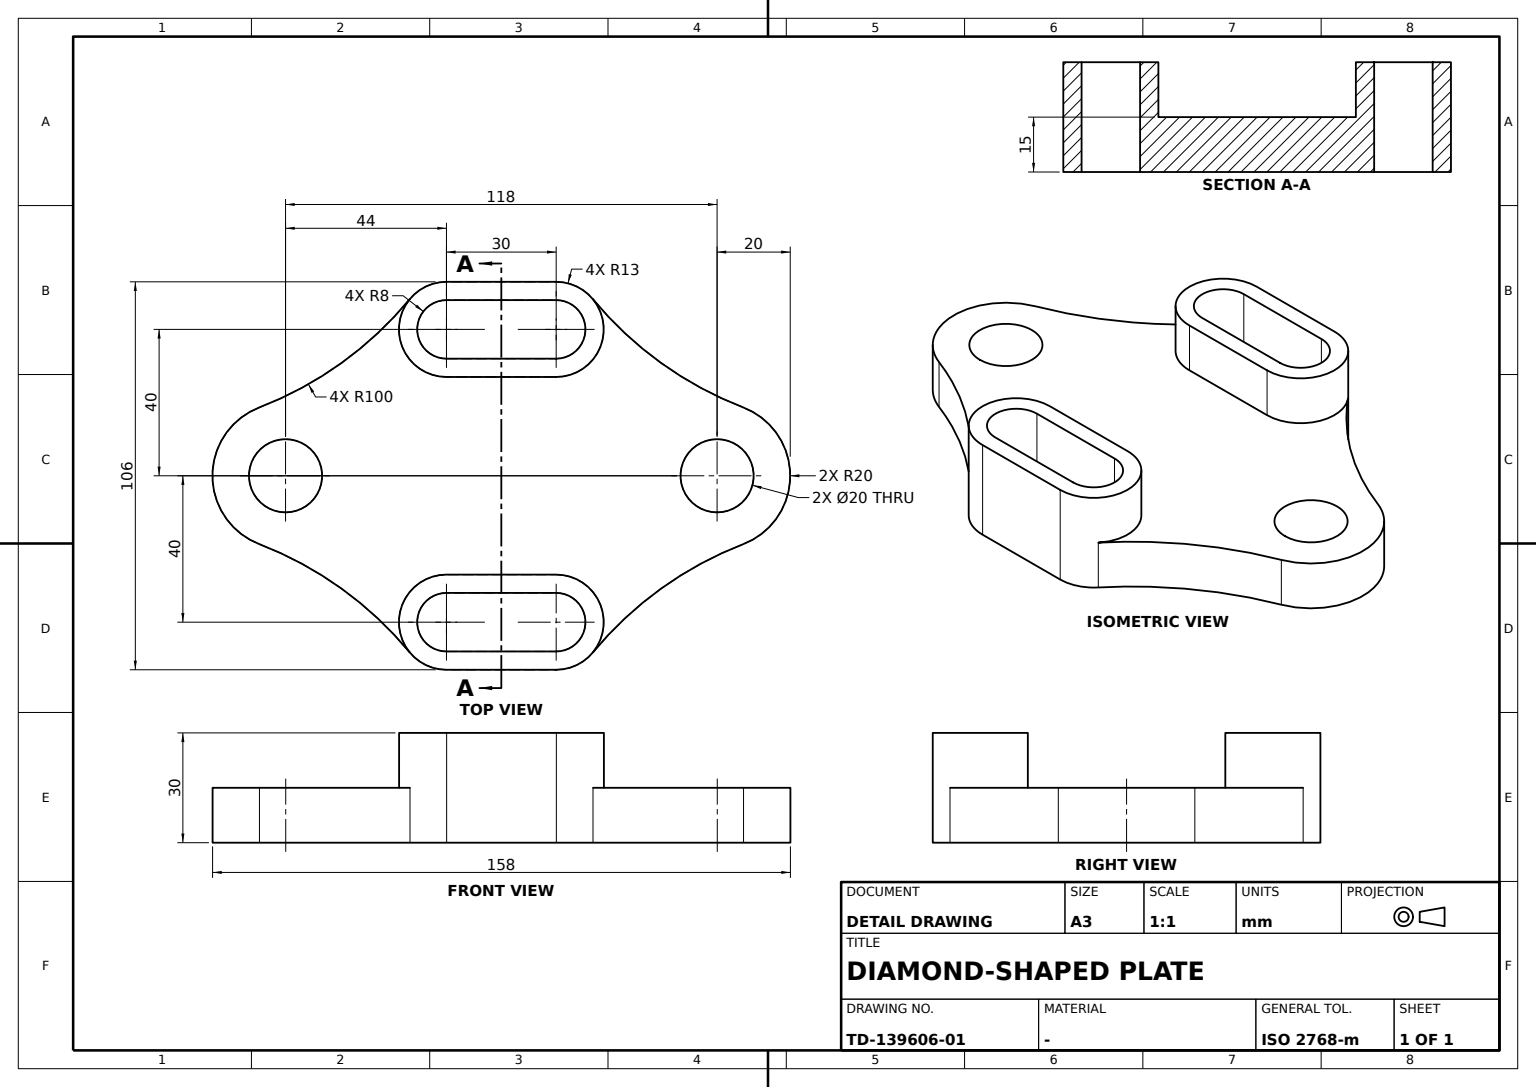
ISO-10303-21;
HEADER;
FILE_DESCRIPTION((''),'2;1');
FILE_NAME('','',(''),(''),'','','');
FILE_SCHEMA(('AUTOMOTIVE_DESIGN'));
ENDSEC;
DATA;
#1=APPLICATION_CONTEXT('');
#2=PRODUCT_CONTEXT('',#1,'mechanical');
#3=PRODUCT('','','',(#2));
#4=PRODUCT_DEFINITION_FORMATION('','',#3);
#5=PRODUCT_DEFINITION_CONTEXT('',#1,'design');
#6=PRODUCT_DEFINITION('','',#4,#5);
#7=PRODUCT_DEFINITION_SHAPE('','',#6);
#8=(LENGTH_UNIT()NAMED_UNIT(*)SI_UNIT(.MILLI.,.METRE.));
#9=(NAMED_UNIT(*)PLANE_ANGLE_UNIT()SI_UNIT($,.RADIAN.));
#10=(NAMED_UNIT(*)SI_UNIT($,.STERADIAN.)SOLID_ANGLE_UNIT());
#11=UNCERTAINTY_MEASURE_WITH_UNIT(LENGTH_MEASURE(0.005),#8,'distance_accuracy_value','');
#12=(GEOMETRIC_REPRESENTATION_CONTEXT(3)GLOBAL_UNCERTAINTY_ASSIGNED_CONTEXT((#11))GLOBAL_UNIT_ASSIGNED_CONTEXT((#8,#9,#10))REPRESENTATION_CONTEXT('',''));
#13=CARTESIAN_POINT('',(-32.,-15.,-15.));
#14=VERTEX_POINT('',#13);
#15=CARTESIAN_POINT('',(-32.,15.,-15.));
#16=VERTEX_POINT('',#15);
#17=DIRECTION('',(0.,1.,0.));
#18=VECTOR('',#17,1000.);
#19=LINE('',#15,#18);
#20=EDGE_CURVE('',#14,#16,#19,.T.);
#21=ORIENTED_EDGE('',*,*,#20,.F.);
#22=CARTESIAN_POINT('',(-32.,-15.,15.));
#23=VERTEX_POINT('',#22);
#24=CARTESIAN_POINT('',(-32.,-15.,7.5));
#25=DIRECTION('',(0.,0.,1.));
#26=VECTOR('',#25,1000.);
#27=LINE('',#24,#26);
#28=EDGE_CURVE('',#23,#14,#27,.F.);
#29=ORIENTED_EDGE('',*,*,#28,.F.);
#30=CARTESIAN_POINT('',(-32.,15.,15.));
#31=VERTEX_POINT('',#30);
#32=CARTESIAN_POINT('',(-32.,0.,15.));
#33=DIRECTION('',(0.,-1.,0.));
#34=VECTOR('',#33,1000.);
#35=LINE('',#32,#34);
#36=EDGE_CURVE('',#31,#23,#35,.T.);
#37=ORIENTED_EDGE('',*,*,#36,.F.);
#38=CARTESIAN_POINT('',(-32.,15.,7.5));
#39=LINE('',#38,#26);
#40=EDGE_CURVE('',#31,#16,#39,.F.);
#41=ORIENTED_EDGE('',*,*,#40,.T.);
#42=EDGE_LOOP('',(#21,#29,#37,#41));
#43=FACE_BOUND('',#42,.T.);
#44=CARTESIAN_POINT('',(-32.,15.,0.));
#45=DIRECTION('',(-1.,0.,0.));
#46=AXIS2_PLACEMENT_3D('',#44,#45,#33);
#47=PLANE('',#46);
#48=ADVANCED_FACE('',(#43),#47,.T.);
#49=CARTESIAN_POINT('',(-48.28249871,-25.01999078,0.));
#50=VERTEX_POINT('',#49);
#51=CARTESIAN_POINT('',(-48.28249871,-25.01999078,-15.));
#52=VERTEX_POINT('',#51);
#53=CARTESIAN_POINT('',(-48.28249871,-25.01999078,-7.5));
#54=LINE('',#53,#26);
#55=EDGE_CURVE('',#50,#52,#54,.F.);
#56=ORIENTED_EDGE('',*,*,#55,.T.);
#57=CARTESIAN_POINT('',(-18.6656712,-66.18280715,-15.));
#58=VERTEX_POINT('',#57);
#59=CARTESIAN_POINT('',(-111.99402721,-102.09684292,-15.));
#60=DIRECTION('',(1.,0.,0.));
#61=AXIS2_PLACEMENT_3D('',#59,#25,#60);
#62=CIRCLE('',#61,100.);
#63=EDGE_CURVE('',#58,#52,#62,.T.);
#64=ORIENTED_EDGE('',*,*,#63,.F.);
#65=CARTESIAN_POINT('',(-18.6656712,-66.18280715,0.));
#66=VERTEX_POINT('',#65);
#67=CARTESIAN_POINT('',(-18.6656712,-66.18280715,-7.5));
#68=LINE('',#67,#26);
#69=EDGE_CURVE('',#66,#58,#68,.F.);
#70=ORIENTED_EDGE('',*,*,#69,.F.);
#71=CARTESIAN_POINT('',(-111.99402721,-102.09684292,0.));
#72=AXIS2_PLACEMENT_3D('',#71,#25,#60);
#73=CIRCLE('',#72,100.);
#74=EDGE_CURVE('',#66,#50,#73,.T.);
#75=ORIENTED_EDGE('',*,*,#74,.T.);
#76=EDGE_LOOP('',(#56,#64,#70,#75));
#77=FACE_BOUND('',#76,.T.);
#78=CARTESIAN_POINT('',(-111.99402721,-102.09684292,-7.5));
#79=AXIS2_PLACEMENT_3D('',#78,#25,#60);
#80=CYLINDRICAL_SURFACE('',#79,100.);
#81=ADVANCED_FACE('',(#77),#80,.F.);
#82=CARTESIAN_POINT('',(10.,-59.,-15.));
#83=VERTEX_POINT('',#82);
#84=CARTESIAN_POINT('',(0.,-59.,-15.));
#85=AXIS2_PLACEMENT_3D('',#84,#25,#60);
#86=CIRCLE('',#85,10.);
#87=EDGE_CURVE('',#83,#83,#86,.T.);
#88=ORIENTED_EDGE('',*,*,#87,.F.);
#89=EDGE_LOOP('',(#88));
#90=FACE_BOUND('',#89,.T.);
#91=CARTESIAN_POINT('',(10.,-59.,0.));
#92=VERTEX_POINT('',#91);
#93=CARTESIAN_POINT('',(0.,-59.,0.));
#94=AXIS2_PLACEMENT_3D('',#93,#25,#60);
#95=CIRCLE('',#94,10.);
#96=EDGE_CURVE('',#92,#92,#95,.T.);
#97=ORIENTED_EDGE('',*,*,#96,.T.);
#98=EDGE_LOOP('',(#97));
#99=FACE_BOUND('',#98,.T.);
#100=CARTESIAN_POINT('',(0.,-59.,-7.5));
#101=AXIS2_PLACEMENT_3D('',#100,#25,#60);
#102=CYLINDRICAL_SURFACE('',#101,10.);
#103=ADVANCED_FACE('',(#90,#99),#102,.F.);
#104=CARTESIAN_POINT('',(48.28249871,-25.01999078,0.));
#105=VERTEX_POINT('',#104);
#106=CARTESIAN_POINT('',(18.6656712,-66.18280715,0.));
#107=VERTEX_POINT('',#106);
#108=CARTESIAN_POINT('',(111.99402721,-102.09684292,0.));
#109=AXIS2_PLACEMENT_3D('',#108,#25,#60);
#110=CIRCLE('',#109,100.);
#111=EDGE_CURVE('',#105,#107,#110,.T.);
#112=ORIENTED_EDGE('',*,*,#111,.T.);
#113=CARTESIAN_POINT('',(18.6656712,-66.18280715,-15.));
#114=VERTEX_POINT('',#113);
#115=CARTESIAN_POINT('',(18.6656712,-66.18280715,-7.5));
#116=LINE('',#115,#26);
#117=EDGE_CURVE('',#107,#114,#116,.F.);
#118=ORIENTED_EDGE('',*,*,#117,.T.);
#119=CARTESIAN_POINT('',(48.28249871,-25.01999078,-15.));
#120=VERTEX_POINT('',#119);
#121=CARTESIAN_POINT('',(111.99402721,-102.09684292,-15.));
#122=AXIS2_PLACEMENT_3D('',#121,#25,#60);
#123=CIRCLE('',#122,100.);
#124=EDGE_CURVE('',#120,#114,#123,.T.);
#125=ORIENTED_EDGE('',*,*,#124,.F.);
#126=CARTESIAN_POINT('',(48.28249871,-25.01999078,-7.5));
#127=LINE('',#126,#26);
#128=EDGE_CURVE('',#105,#120,#127,.F.);
#129=ORIENTED_EDGE('',*,*,#128,.F.);
#130=EDGE_LOOP('',(#112,#118,#125,#129));
#131=FACE_BOUND('',#130,.T.);
#132=CARTESIAN_POINT('',(111.99402721,-102.09684292,-7.5));
#133=AXIS2_PLACEMENT_3D('',#132,#25,#60);
#134=CYLINDRICAL_SURFACE('',#133,100.);
#135=ADVANCED_FACE('',(#131),#134,.F.);
#136=CARTESIAN_POINT('',(48.,15.,15.));
#137=VERTEX_POINT('',#136);
#138=CARTESIAN_POINT('',(48.,15.,-15.));
#139=VERTEX_POINT('',#138);
#140=CARTESIAN_POINT('',(48.,15.,7.5));
#141=LINE('',#140,#26);
#142=EDGE_CURVE('',#137,#139,#141,.F.);
#143=ORIENTED_EDGE('',*,*,#142,.T.);
#144=CARTESIAN_POINT('',(48.,-15.,-15.));
#145=VERTEX_POINT('',#144);
#146=LINE('',#138,#18);
#147=EDGE_CURVE('',#145,#139,#146,.T.);
#148=ORIENTED_EDGE('',*,*,#147,.F.);
#149=CARTESIAN_POINT('',(48.,-15.,15.));
#150=VERTEX_POINT('',#149);
#151=CARTESIAN_POINT('',(48.,-15.,7.5));
#152=LINE('',#151,#26);
#153=EDGE_CURVE('',#150,#145,#152,.F.);
#154=ORIENTED_EDGE('',*,*,#153,.F.);
#155=CARTESIAN_POINT('',(48.,0.,15.));
#156=LINE('',#155,#34);
#157=EDGE_CURVE('',#137,#150,#156,.T.);
#158=ORIENTED_EDGE('',*,*,#157,.F.);
#159=EDGE_LOOP('',(#143,#148,#154,#158));
#160=FACE_BOUND('',#159,.T.);
#161=CARTESIAN_POINT('',(48.,15.,0.));
#162=AXIS2_PLACEMENT_3D('',#161,#45,#33);
#163=PLANE('',#162);
#164=ADVANCED_FACE('',(#160),#163,.T.);
#165=CARTESIAN_POINT('',(-48.,15.,-15.));
#166=VERTEX_POINT('',#165);
#167=CARTESIAN_POINT('',(-40.,15.,-15.));
#168=AXIS2_PLACEMENT_3D('',#167,#25,#60);
#169=CIRCLE('',#168,8.);
#170=EDGE_CURVE('',#16,#166,#169,.T.);
#171=ORIENTED_EDGE('',*,*,#170,.F.);
#172=ORIENTED_EDGE('',*,*,#40,.F.);
#173=CARTESIAN_POINT('',(-48.,15.,15.));
#174=VERTEX_POINT('',#173);
#175=CARTESIAN_POINT('',(-40.,15.,15.));
#176=AXIS2_PLACEMENT_3D('',#175,#25,#60);
#177=CIRCLE('',#176,8.);
#178=EDGE_CURVE('',#31,#174,#177,.T.);
#179=ORIENTED_EDGE('',*,*,#178,.T.);
#180=CARTESIAN_POINT('',(-48.,15.,7.5));
#181=LINE('',#180,#26);
#182=EDGE_CURVE('',#174,#166,#181,.F.);
#183=ORIENTED_EDGE('',*,*,#182,.T.);
#184=EDGE_LOOP('',(#171,#172,#179,#183));
#185=FACE_BOUND('',#184,.T.);
#186=CARTESIAN_POINT('',(-40.,15.,7.5));
#187=AXIS2_PLACEMENT_3D('',#186,#25,#60);
#188=CYLINDRICAL_SURFACE('',#187,8.);
#189=ADVANCED_FACE('',(#185),#188,.F.);
#190=ORIENTED_EDGE('',*,*,#142,.F.);
#191=CARTESIAN_POINT('',(32.,15.,15.));
#192=VERTEX_POINT('',#191);
#193=CARTESIAN_POINT('',(40.,15.,15.));
#194=AXIS2_PLACEMENT_3D('',#193,#25,#60);
#195=CIRCLE('',#194,8.);
#196=EDGE_CURVE('',#137,#192,#195,.T.);
#197=ORIENTED_EDGE('',*,*,#196,.T.);
#198=CARTESIAN_POINT('',(32.,15.,-15.));
#199=VERTEX_POINT('',#198);
#200=CARTESIAN_POINT('',(32.,15.,7.5));
#201=LINE('',#200,#26);
#202=EDGE_CURVE('',#192,#199,#201,.F.);
#203=ORIENTED_EDGE('',*,*,#202,.T.);
#204=CARTESIAN_POINT('',(40.,15.,-15.));
#205=AXIS2_PLACEMENT_3D('',#204,#25,#60);
#206=CIRCLE('',#205,8.);
#207=EDGE_CURVE('',#139,#199,#206,.T.);
#208=ORIENTED_EDGE('',*,*,#207,.F.);
#209=EDGE_LOOP('',(#190,#197,#203,#208));
#210=FACE_BOUND('',#209,.T.);
#211=CARTESIAN_POINT('',(40.,15.,7.5));
#212=AXIS2_PLACEMENT_3D('',#211,#25,#60);
#213=CYLINDRICAL_SURFACE('',#212,8.);
#214=ADVANCED_FACE('',(#210),#213,.F.);
#215=CARTESIAN_POINT('',(-48.,-15.,-15.));
#216=VERTEX_POINT('',#215);
#217=LINE('',#215,#34);
#218=EDGE_CURVE('',#166,#216,#217,.T.);
#219=ORIENTED_EDGE('',*,*,#218,.F.);
#220=ORIENTED_EDGE('',*,*,#182,.F.);
#221=CARTESIAN_POINT('',(-48.,-15.,15.));
#222=VERTEX_POINT('',#221);
#223=CARTESIAN_POINT('',(-48.,0.,15.));
#224=LINE('',#223,#18);
#225=EDGE_CURVE('',#222,#174,#224,.T.);
#226=ORIENTED_EDGE('',*,*,#225,.F.);
#227=CARTESIAN_POINT('',(-48.,-15.,7.5));
#228=LINE('',#227,#26);
#229=EDGE_CURVE('',#222,#216,#228,.F.);
#230=ORIENTED_EDGE('',*,*,#229,.T.);
#231=EDGE_LOOP('',(#219,#220,#226,#230));
#232=FACE_BOUND('',#231,.T.);
#233=CARTESIAN_POINT('',(-48.,-15.,0.));
#234=AXIS2_PLACEMENT_3D('',#233,#60,#17);
#235=PLANE('',#234);
#236=ADVANCED_FACE('',(#232),#235,.T.);
#237=CARTESIAN_POINT('',(53.,-15.,15.));
#238=VERTEX_POINT('',#237);
#239=CARTESIAN_POINT('',(53.,-15.,-15.));
#240=VERTEX_POINT('',#239);
#241=CARTESIAN_POINT('',(53.,-15.,-7.5));
#242=LINE('',#241,#26);
#243=EDGE_CURVE('',#238,#240,#242,.F.);
#244=ORIENTED_EDGE('',*,*,#243,.T.);
#245=CARTESIAN_POINT('',(53.,15.,-15.));
#246=VERTEX_POINT('',#245);
#247=LINE('',#245,#34);
#248=EDGE_CURVE('',#246,#240,#247,.T.);
#249=ORIENTED_EDGE('',*,*,#248,.F.);
#250=CARTESIAN_POINT('',(53.,15.,15.));
#251=VERTEX_POINT('',#250);
#252=CARTESIAN_POINT('',(53.,15.,7.5));
#253=LINE('',#252,#26);
#254=EDGE_CURVE('',#251,#246,#253,.F.);
#255=ORIENTED_EDGE('',*,*,#254,.F.);
#256=LINE('',#250,#34);
#257=EDGE_CURVE('',#251,#238,#256,.T.);
#258=ORIENTED_EDGE('',*,*,#257,.T.);
#259=EDGE_LOOP('',(#244,#249,#255,#258));
#260=FACE_BOUND('',#259,.T.);
#261=CARTESIAN_POINT('',(53.,15.,0.));
#262=AXIS2_PLACEMENT_3D('',#261,#60,#33);
#263=PLANE('',#262);
#264=ADVANCED_FACE('',(#260),#263,.T.);
#265=CARTESIAN_POINT('',(10.,59.,-15.));
#266=VERTEX_POINT('',#265);
#267=CARTESIAN_POINT('',(0.,59.,-15.));
#268=AXIS2_PLACEMENT_3D('',#267,#25,#60);
#269=CIRCLE('',#268,10.);
#270=EDGE_CURVE('',#266,#266,#269,.T.);
#271=ORIENTED_EDGE('',*,*,#270,.F.);
#272=EDGE_LOOP('',(#271));
#273=FACE_BOUND('',#272,.T.);
#274=CARTESIAN_POINT('',(10.,59.,0.));
#275=VERTEX_POINT('',#274);
#276=CARTESIAN_POINT('',(0.,59.,0.));
#277=AXIS2_PLACEMENT_3D('',#276,#25,#60);
#278=CIRCLE('',#277,10.);
#279=EDGE_CURVE('',#275,#275,#278,.T.);
#280=ORIENTED_EDGE('',*,*,#279,.T.);
#281=EDGE_LOOP('',(#280));
#282=FACE_BOUND('',#281,.T.);
#283=CARTESIAN_POINT('',(0.,59.,-7.5));
#284=AXIS2_PLACEMENT_3D('',#283,#25,#60);
#285=CYLINDRICAL_SURFACE('',#284,10.);
#286=ADVANCED_FACE('',(#273,#282),#285,.F.);
#287=CARTESIAN_POINT('',(32.,-15.,-15.));
#288=VERTEX_POINT('',#287);
#289=LINE('',#287,#34);
#290=EDGE_CURVE('',#199,#288,#289,.T.);
#291=ORIENTED_EDGE('',*,*,#290,.F.);
#292=ORIENTED_EDGE('',*,*,#202,.F.);
#293=CARTESIAN_POINT('',(32.,-15.,15.));
#294=VERTEX_POINT('',#293);
#295=CARTESIAN_POINT('',(32.,0.,15.));
#296=LINE('',#295,#18);
#297=EDGE_CURVE('',#294,#192,#296,.T.);
#298=ORIENTED_EDGE('',*,*,#297,.F.);
#299=CARTESIAN_POINT('',(32.,-15.,7.5));
#300=LINE('',#299,#26);
#301=EDGE_CURVE('',#294,#288,#300,.F.);
#302=ORIENTED_EDGE('',*,*,#301,.T.);
#303=EDGE_LOOP('',(#291,#292,#298,#302));
#304=FACE_BOUND('',#303,.T.);
#305=CARTESIAN_POINT('',(32.,-15.,0.));
#306=AXIS2_PLACEMENT_3D('',#305,#60,#17);
#307=PLANE('',#306);
#308=ADVANCED_FACE('',(#304),#307,.T.);
#309=CARTESIAN_POINT('',(-53.,-15.,15.));
#310=VERTEX_POINT('',#309);
#311=CARTESIAN_POINT('',(-53.,-15.,-15.));
#312=VERTEX_POINT('',#311);
#313=CARTESIAN_POINT('',(-53.,-15.,-7.5));
#314=LINE('',#313,#26);
#315=EDGE_CURVE('',#310,#312,#314,.F.);
#316=ORIENTED_EDGE('',*,*,#315,.F.);
#317=CARTESIAN_POINT('',(-53.,15.,15.));
#318=VERTEX_POINT('',#317);
#319=LINE('',#309,#18);
#320=EDGE_CURVE('',#310,#318,#319,.T.);
#321=ORIENTED_EDGE('',*,*,#320,.T.);
#322=CARTESIAN_POINT('',(-53.,15.,-15.));
#323=VERTEX_POINT('',#322);
#324=CARTESIAN_POINT('',(-53.,15.,-7.5));
#325=LINE('',#324,#26);
#326=EDGE_CURVE('',#318,#323,#325,.F.);
#327=ORIENTED_EDGE('',*,*,#326,.T.);
#328=LINE('',#311,#18);
#329=EDGE_CURVE('',#312,#323,#328,.T.);
#330=ORIENTED_EDGE('',*,*,#329,.F.);
#331=EDGE_LOOP('',(#316,#321,#327,#330));
#332=FACE_BOUND('',#331,.T.);
#333=CARTESIAN_POINT('',(-53.,-15.,0.));
#334=AXIS2_PLACEMENT_3D('',#333,#45,#17);
#335=PLANE('',#334);
#336=ADVANCED_FACE('',(#332),#335,.T.);
#337=CARTESIAN_POINT('',(40.,-15.,-15.));
#338=AXIS2_PLACEMENT_3D('',#337,#25,#60);
#339=CIRCLE('',#338,13.);
#340=EDGE_CURVE('',#120,#240,#339,.T.);
#341=ORIENTED_EDGE('',*,*,#340,.T.);
#342=ORIENTED_EDGE('',*,*,#243,.F.);
#343=CARTESIAN_POINT('',(27.,-15.,15.));
#344=VERTEX_POINT('',#343);
#345=CARTESIAN_POINT('',(40.,-15.,15.));
#346=AXIS2_PLACEMENT_3D('',#345,#25,#60);
#347=CIRCLE('',#346,13.);
#348=EDGE_CURVE('',#344,#238,#347,.T.);
#349=ORIENTED_EDGE('',*,*,#348,.F.);
#350=CARTESIAN_POINT('',(27.,-15.,0.));
#351=VERTEX_POINT('',#350);
#352=CARTESIAN_POINT('',(27.,-15.,-7.5));
#353=LINE('',#352,#26);
#354=EDGE_CURVE('',#351,#344,#353,.T.);
#355=ORIENTED_EDGE('',*,*,#354,.F.);
#356=CARTESIAN_POINT('',(40.,-15.,0.));
#357=AXIS2_PLACEMENT_3D('',#356,#25,#60);
#358=CIRCLE('',#357,13.);
#359=EDGE_CURVE('',#351,#105,#358,.T.);
#360=ORIENTED_EDGE('',*,*,#359,.T.);
#361=ORIENTED_EDGE('',*,*,#128,.T.);
#362=EDGE_LOOP('',(#341,#342,#349,#355,#360,#361));
#363=FACE_BOUND('',#362,.T.);
#364=CARTESIAN_POINT('',(40.,-15.,-7.5));
#365=AXIS2_PLACEMENT_3D('',#364,#25,#60);
#366=CYLINDRICAL_SURFACE('',#365,13.);
#367=ADVANCED_FACE('',(#363),#366,.T.);
#368=CARTESIAN_POINT('',(18.6656712,66.18280715,-15.));
#369=VERTEX_POINT('',#368);
#370=CARTESIAN_POINT('',(48.28249871,25.01999078,-15.));
#371=VERTEX_POINT('',#370);
#372=CARTESIAN_POINT('',(111.99402721,102.09684292,-15.));
#373=AXIS2_PLACEMENT_3D('',#372,#25,#60);
#374=CIRCLE('',#373,100.);
#375=EDGE_CURVE('',#369,#371,#374,.T.);
#376=ORIENTED_EDGE('',*,*,#375,.F.);
#377=CARTESIAN_POINT('',(18.6656712,66.18280715,0.));
#378=VERTEX_POINT('',#377);
#379=CARTESIAN_POINT('',(18.6656712,66.18280715,-7.5));
#380=LINE('',#379,#26);
#381=EDGE_CURVE('',#378,#369,#380,.F.);
#382=ORIENTED_EDGE('',*,*,#381,.F.);
#383=CARTESIAN_POINT('',(48.28249871,25.01999078,0.));
#384=VERTEX_POINT('',#383);
#385=CARTESIAN_POINT('',(111.99402721,102.09684292,0.));
#386=AXIS2_PLACEMENT_3D('',#385,#25,#60);
#387=CIRCLE('',#386,100.);
#388=EDGE_CURVE('',#378,#384,#387,.T.);
#389=ORIENTED_EDGE('',*,*,#388,.T.);
#390=CARTESIAN_POINT('',(48.28249871,25.01999078,-7.5));
#391=LINE('',#390,#26);
#392=EDGE_CURVE('',#384,#371,#391,.F.);
#393=ORIENTED_EDGE('',*,*,#392,.T.);
#394=EDGE_LOOP('',(#376,#382,#389,#393));
#395=FACE_BOUND('',#394,.T.);
#396=CARTESIAN_POINT('',(111.99402721,102.09684292,-7.5));
#397=AXIS2_PLACEMENT_3D('',#396,#25,#60);
#398=CYLINDRICAL_SURFACE('',#397,100.);
#399=ADVANCED_FACE('',(#395),#398,.F.);
#400=CARTESIAN_POINT('',(-48.28249871,25.01999078,0.));
#401=VERTEX_POINT('',#400);
#402=CARTESIAN_POINT('',(-48.28249871,25.01999078,-15.));
#403=VERTEX_POINT('',#402);
#404=CARTESIAN_POINT('',(-48.28249871,25.01999078,-7.5));
#405=LINE('',#404,#26);
#406=EDGE_CURVE('',#401,#403,#405,.F.);
#407=ORIENTED_EDGE('',*,*,#406,.F.);
#408=CARTESIAN_POINT('',(-18.6656712,66.18280715,0.));
#409=VERTEX_POINT('',#408);
#410=CARTESIAN_POINT('',(-111.99402721,102.09684292,0.));
#411=AXIS2_PLACEMENT_3D('',#410,#25,#60);
#412=CIRCLE('',#411,100.);
#413=EDGE_CURVE('',#401,#409,#412,.T.);
#414=ORIENTED_EDGE('',*,*,#413,.T.);
#415=CARTESIAN_POINT('',(-18.6656712,66.18280715,-15.));
#416=VERTEX_POINT('',#415);
#417=CARTESIAN_POINT('',(-18.6656712,66.18280715,-7.5));
#418=LINE('',#417,#26);
#419=EDGE_CURVE('',#409,#416,#418,.F.);
#420=ORIENTED_EDGE('',*,*,#419,.T.);
#421=CARTESIAN_POINT('',(-111.99402721,102.09684292,-15.));
#422=AXIS2_PLACEMENT_3D('',#421,#25,#60);
#423=CIRCLE('',#422,100.);
#424=EDGE_CURVE('',#403,#416,#423,.T.);
#425=ORIENTED_EDGE('',*,*,#424,.F.);
#426=EDGE_LOOP('',(#407,#414,#420,#425));
#427=FACE_BOUND('',#426,.T.);
#428=CARTESIAN_POINT('',(-111.99402721,102.09684292,-7.5));
#429=AXIS2_PLACEMENT_3D('',#428,#25,#60);
#430=CYLINDRICAL_SURFACE('',#429,100.);
#431=ADVANCED_FACE('',(#427),#430,.F.);
#432=CARTESIAN_POINT('',(27.,15.,15.));
#433=VERTEX_POINT('',#432);
#434=CARTESIAN_POINT('',(27.,0.,15.));
#435=LINE('',#434,#18);
#436=EDGE_CURVE('',#344,#433,#435,.T.);
#437=ORIENTED_EDGE('',*,*,#436,.T.);
#438=CARTESIAN_POINT('',(27.,15.,0.));
#439=VERTEX_POINT('',#438);
#440=CARTESIAN_POINT('',(27.,15.,7.5));
#441=LINE('',#440,#26);
#442=EDGE_CURVE('',#439,#433,#441,.T.);
#443=ORIENTED_EDGE('',*,*,#442,.F.);
#444=CARTESIAN_POINT('',(27.,0.,0.));
#445=LINE('',#444,#18);
#446=EDGE_CURVE('',#351,#439,#445,.T.);
#447=ORIENTED_EDGE('',*,*,#446,.F.);
#448=ORIENTED_EDGE('',*,*,#354,.T.);
#449=EDGE_LOOP('',(#437,#443,#447,#448));
#450=FACE_BOUND('',#449,.T.);
#451=AXIS2_PLACEMENT_3D('',#350,#60,#17);
#452=PLANE('',#451);
#453=ADVANCED_FACE('',(#450),#452,.F.);
#454=CARTESIAN_POINT('',(-27.,15.,15.));
#455=VERTEX_POINT('',#454);
#456=CIRCLE('',#176,13.);
#457=EDGE_CURVE('',#455,#318,#456,.T.);
#458=ORIENTED_EDGE('',*,*,#457,.T.);
#459=ORIENTED_EDGE('',*,*,#320,.F.);
#460=CARTESIAN_POINT('',(-27.,-15.,15.));
#461=VERTEX_POINT('',#460);
#462=CARTESIAN_POINT('',(-40.,-15.,15.));
#463=AXIS2_PLACEMENT_3D('',#462,#25,#60);
#464=CIRCLE('',#463,13.);
#465=EDGE_CURVE('',#310,#461,#464,.T.);
#466=ORIENTED_EDGE('',*,*,#465,.T.);
#467=CARTESIAN_POINT('',(-27.,0.,15.));
#468=LINE('',#467,#34);
#469=EDGE_CURVE('',#455,#461,#468,.T.);
#470=ORIENTED_EDGE('',*,*,#469,.F.);
#471=EDGE_LOOP('',(#458,#459,#466,#470));
#472=FACE_BOUND('',#471,.T.);
#473=ORIENTED_EDGE('',*,*,#178,.F.);
#474=ORIENTED_EDGE('',*,*,#36,.T.);
#475=CIRCLE('',#463,8.);
#476=EDGE_CURVE('',#222,#23,#475,.T.);
#477=ORIENTED_EDGE('',*,*,#476,.F.);
#478=ORIENTED_EDGE('',*,*,#225,.T.);
#479=EDGE_LOOP('',(#473,#474,#477,#478));
#480=FACE_BOUND('',#479,.T.);
#481=CARTESIAN_POINT('',(0.,0.,15.));
#482=AXIS2_PLACEMENT_3D('',#481,#25,#60);
#483=PLANE('',#482);
#484=ADVANCED_FACE('',(#472,#480),#483,.T.);
#485=CIRCLE('',#338,8.);
#486=EDGE_CURVE('',#288,#145,#485,.T.);
#487=ORIENTED_EDGE('',*,*,#486,.F.);
#488=ORIENTED_EDGE('',*,*,#301,.F.);
#489=CIRCLE('',#346,8.);
#490=EDGE_CURVE('',#294,#150,#489,.T.);
#491=ORIENTED_EDGE('',*,*,#490,.T.);
#492=ORIENTED_EDGE('',*,*,#153,.T.);
#493=EDGE_LOOP('',(#487,#488,#491,#492));
#494=FACE_BOUND('',#493,.T.);
#495=CARTESIAN_POINT('',(40.,-15.,7.5));
#496=AXIS2_PLACEMENT_3D('',#495,#25,#60);
#497=CYLINDRICAL_SURFACE('',#496,8.);
#498=ADVANCED_FACE('',(#494),#497,.F.);
#499=ORIENTED_EDGE('',*,*,#279,.F.);
#500=EDGE_LOOP('',(#499));
#501=FACE_BOUND('',#500,.T.);
#502=ORIENTED_EDGE('',*,*,#96,.F.);
#503=EDGE_LOOP('',(#502));
#504=FACE_BOUND('',#503,.T.);
#505=CIRCLE('',#94,20.);
#506=EDGE_CURVE('',#66,#107,#505,.T.);
#507=ORIENTED_EDGE('',*,*,#506,.T.);
#508=ORIENTED_EDGE('',*,*,#111,.F.);
#509=ORIENTED_EDGE('',*,*,#359,.F.);
#510=ORIENTED_EDGE('',*,*,#446,.T.);
#511=CARTESIAN_POINT('',(40.,15.,0.));
#512=AXIS2_PLACEMENT_3D('',#511,#25,#60);
#513=CIRCLE('',#512,13.);
#514=EDGE_CURVE('',#384,#439,#513,.T.);
#515=ORIENTED_EDGE('',*,*,#514,.F.);
#516=ORIENTED_EDGE('',*,*,#388,.F.);
#517=CIRCLE('',#277,20.);
#518=EDGE_CURVE('',#378,#409,#517,.T.);
#519=ORIENTED_EDGE('',*,*,#518,.T.);
#520=ORIENTED_EDGE('',*,*,#413,.F.);
#521=CARTESIAN_POINT('',(-27.,15.,0.));
#522=VERTEX_POINT('',#521);
#523=CARTESIAN_POINT('',(-40.,15.,0.));
#524=AXIS2_PLACEMENT_3D('',#523,#25,#60);
#525=CIRCLE('',#524,13.);
#526=EDGE_CURVE('',#522,#401,#525,.T.);
#527=ORIENTED_EDGE('',*,*,#526,.F.);
#528=CARTESIAN_POINT('',(-27.,-15.,0.));
#529=VERTEX_POINT('',#528);
#530=CARTESIAN_POINT('',(-27.,0.,0.));
#531=LINE('',#530,#34);
#532=EDGE_CURVE('',#522,#529,#531,.T.);
#533=ORIENTED_EDGE('',*,*,#532,.T.);
#534=CARTESIAN_POINT('',(-40.,-15.,0.));
#535=AXIS2_PLACEMENT_3D('',#534,#25,#60);
#536=CIRCLE('',#535,13.);
#537=EDGE_CURVE('',#50,#529,#536,.T.);
#538=ORIENTED_EDGE('',*,*,#537,.F.);
#539=ORIENTED_EDGE('',*,*,#74,.F.);
#540=EDGE_LOOP('',(#507,#508,#509,#510,#515,#516,#519,#520,#527,#533,#538,#539));
#541=FACE_BOUND('',#540,.T.);
#542=CARTESIAN_POINT('',(0.,0.,0.));
#543=AXIS2_PLACEMENT_3D('',#542,#25,#60);
#544=PLANE('',#543);
#545=ADVANCED_FACE('',(#501,#504,#541),#544,.T.);
#546=ORIENTED_EDGE('',*,*,#490,.F.);
#547=ORIENTED_EDGE('',*,*,#297,.T.);
#548=ORIENTED_EDGE('',*,*,#196,.F.);
#549=ORIENTED_EDGE('',*,*,#157,.T.);
#550=EDGE_LOOP('',(#546,#547,#548,#549));
#551=FACE_BOUND('',#550,.T.);
#552=ORIENTED_EDGE('',*,*,#436,.F.);
#553=ORIENTED_EDGE('',*,*,#348,.T.);
#554=ORIENTED_EDGE('',*,*,#257,.F.);
#555=CIRCLE('',#194,13.);
#556=EDGE_CURVE('',#251,#433,#555,.T.);
#557=ORIENTED_EDGE('',*,*,#556,.T.);
#558=EDGE_LOOP('',(#552,#553,#554,#557));
#559=FACE_BOUND('',#558,.T.);
#560=ADVANCED_FACE('',(#551,#559),#483,.T.);
#561=ORIENTED_EDGE('',*,*,#87,.T.);
#562=EDGE_LOOP('',(#561));
#563=FACE_BOUND('',#562,.T.);
#564=ORIENTED_EDGE('',*,*,#20,.T.);
#565=ORIENTED_EDGE('',*,*,#170,.T.);
#566=ORIENTED_EDGE('',*,*,#218,.T.);
#567=CARTESIAN_POINT('',(-40.,-15.,-15.));
#568=AXIS2_PLACEMENT_3D('',#567,#25,#60);
#569=CIRCLE('',#568,8.);
#570=EDGE_CURVE('',#216,#14,#569,.T.);
#571=ORIENTED_EDGE('',*,*,#570,.T.);
#572=EDGE_LOOP('',(#564,#565,#566,#571));
#573=FACE_BOUND('',#572,.T.);
#574=ORIENTED_EDGE('',*,*,#290,.T.);
#575=ORIENTED_EDGE('',*,*,#486,.T.);
#576=ORIENTED_EDGE('',*,*,#147,.T.);
#577=ORIENTED_EDGE('',*,*,#207,.T.);
#578=EDGE_LOOP('',(#574,#575,#576,#577));
#579=FACE_BOUND('',#578,.T.);
#580=ORIENTED_EDGE('',*,*,#270,.T.);
#581=EDGE_LOOP('',(#580));
#582=FACE_BOUND('',#581,.T.);
#583=ORIENTED_EDGE('',*,*,#248,.T.);
#584=ORIENTED_EDGE('',*,*,#340,.F.);
#585=ORIENTED_EDGE('',*,*,#124,.T.);
#586=CIRCLE('',#85,20.);
#587=EDGE_CURVE('',#58,#114,#586,.T.);
#588=ORIENTED_EDGE('',*,*,#587,.F.);
#589=ORIENTED_EDGE('',*,*,#63,.T.);
#590=CIRCLE('',#568,13.);
#591=EDGE_CURVE('',#312,#52,#590,.T.);
#592=ORIENTED_EDGE('',*,*,#591,.F.);
#593=ORIENTED_EDGE('',*,*,#329,.T.);
#594=CIRCLE('',#168,13.);
#595=EDGE_CURVE('',#403,#323,#594,.T.);
#596=ORIENTED_EDGE('',*,*,#595,.F.);
#597=ORIENTED_EDGE('',*,*,#424,.T.);
#598=CIRCLE('',#268,20.);
#599=EDGE_CURVE('',#369,#416,#598,.T.);
#600=ORIENTED_EDGE('',*,*,#599,.F.);
#601=ORIENTED_EDGE('',*,*,#375,.T.);
#602=CIRCLE('',#205,13.);
#603=EDGE_CURVE('',#246,#371,#602,.T.);
#604=ORIENTED_EDGE('',*,*,#603,.F.);
#605=EDGE_LOOP('',(#583,#584,#585,#588,#589,#592,#593,#596,#597,#600,#601,#604));
#606=FACE_BOUND('',#605,.T.);
#607=CARTESIAN_POINT('',(0.,0.,-15.));
#608=AXIS2_PLACEMENT_3D('',#607,#25,#60);
#609=PLANE('',#608);
#610=ADVANCED_FACE('',(#563,#573,#579,#582,#606),#609,.F.);
#611=ORIENTED_EDGE('',*,*,#506,.F.);
#612=ORIENTED_EDGE('',*,*,#69,.T.);
#613=ORIENTED_EDGE('',*,*,#587,.T.);
#614=ORIENTED_EDGE('',*,*,#117,.F.);
#615=EDGE_LOOP('',(#611,#612,#613,#614));
#616=FACE_BOUND('',#615,.T.);
#617=CYLINDRICAL_SURFACE('',#101,20.);
#618=ADVANCED_FACE('',(#616),#617,.T.);
#619=ORIENTED_EDGE('',*,*,#469,.T.);
#620=CARTESIAN_POINT('',(-27.,-15.,-7.5));
#621=LINE('',#620,#26);
#622=EDGE_CURVE('',#529,#461,#621,.T.);
#623=ORIENTED_EDGE('',*,*,#622,.F.);
#624=ORIENTED_EDGE('',*,*,#532,.F.);
#625=CARTESIAN_POINT('',(-27.,15.,-7.5));
#626=LINE('',#625,#26);
#627=EDGE_CURVE('',#522,#455,#626,.T.);
#628=ORIENTED_EDGE('',*,*,#627,.T.);
#629=EDGE_LOOP('',(#619,#623,#624,#628));
#630=FACE_BOUND('',#629,.T.);
#631=AXIS2_PLACEMENT_3D('',#521,#45,#33);
#632=PLANE('',#631);
#633=ADVANCED_FACE('',(#630),#632,.F.);
#634=ORIENTED_EDGE('',*,*,#595,.T.);
#635=ORIENTED_EDGE('',*,*,#326,.F.);
#636=ORIENTED_EDGE('',*,*,#457,.F.);
#637=ORIENTED_EDGE('',*,*,#627,.F.);
#638=ORIENTED_EDGE('',*,*,#526,.T.);
#639=ORIENTED_EDGE('',*,*,#406,.T.);
#640=EDGE_LOOP('',(#634,#635,#636,#637,#638,#639));
#641=FACE_BOUND('',#640,.T.);
#642=CARTESIAN_POINT('',(-40.,15.,-7.5));
#643=AXIS2_PLACEMENT_3D('',#642,#25,#60);
#644=CYLINDRICAL_SURFACE('',#643,13.);
#645=ADVANCED_FACE('',(#641),#644,.T.);
#646=ORIENTED_EDGE('',*,*,#556,.F.);
#647=ORIENTED_EDGE('',*,*,#254,.T.);
#648=ORIENTED_EDGE('',*,*,#603,.T.);
#649=ORIENTED_EDGE('',*,*,#392,.F.);
#650=ORIENTED_EDGE('',*,*,#514,.T.);
#651=ORIENTED_EDGE('',*,*,#442,.T.);
#652=EDGE_LOOP('',(#646,#647,#648,#649,#650,#651));
#653=FACE_BOUND('',#652,.T.);
#654=CYLINDRICAL_SURFACE('',#212,13.);
#655=ADVANCED_FACE('',(#653),#654,.T.);
#656=ORIENTED_EDGE('',*,*,#591,.T.);
#657=ORIENTED_EDGE('',*,*,#55,.F.);
#658=ORIENTED_EDGE('',*,*,#537,.T.);
#659=ORIENTED_EDGE('',*,*,#622,.T.);
#660=ORIENTED_EDGE('',*,*,#465,.F.);
#661=ORIENTED_EDGE('',*,*,#315,.T.);
#662=EDGE_LOOP('',(#656,#657,#658,#659,#660,#661));
#663=FACE_BOUND('',#662,.T.);
#664=CARTESIAN_POINT('',(-40.,-15.,-7.5));
#665=AXIS2_PLACEMENT_3D('',#664,#25,#60);
#666=CYLINDRICAL_SURFACE('',#665,13.);
#667=ADVANCED_FACE('',(#663),#666,.T.);
#668=ORIENTED_EDGE('',*,*,#599,.T.);
#669=ORIENTED_EDGE('',*,*,#419,.F.);
#670=ORIENTED_EDGE('',*,*,#518,.F.);
#671=ORIENTED_EDGE('',*,*,#381,.T.);
#672=EDGE_LOOP('',(#668,#669,#670,#671));
#673=FACE_BOUND('',#672,.T.);
#674=CYLINDRICAL_SURFACE('',#284,20.);
#675=ADVANCED_FACE('',(#673),#674,.T.);
#676=ORIENTED_EDGE('',*,*,#229,.F.);
#677=ORIENTED_EDGE('',*,*,#476,.T.);
#678=ORIENTED_EDGE('',*,*,#28,.T.);
#679=ORIENTED_EDGE('',*,*,#570,.F.);
#680=EDGE_LOOP('',(#676,#677,#678,#679));
#681=FACE_BOUND('',#680,.T.);
#682=CARTESIAN_POINT('',(-40.,-15.,7.5));
#683=AXIS2_PLACEMENT_3D('',#682,#25,#60);
#684=CYLINDRICAL_SURFACE('',#683,8.);
#685=ADVANCED_FACE('',(#681),#684,.F.);
#686=CLOSED_SHELL('',(#48,#81,#103,#135,#164,#189,#214,#236,#264,#286,#308,#336,#367,#399,#431,#453,#484,#498,#545,#560,#610,#618,#633,#645,#655,#667,#675,#685));
#687=MANIFOLD_SOLID_BREP('',#686);
#688=ADVANCED_BREP_SHAPE_REPRESENTATION('',(#687),#12);
#689=SHAPE_DEFINITION_REPRESENTATION(#7,#688);
ENDSEC;
END-ISO-10303-21;
